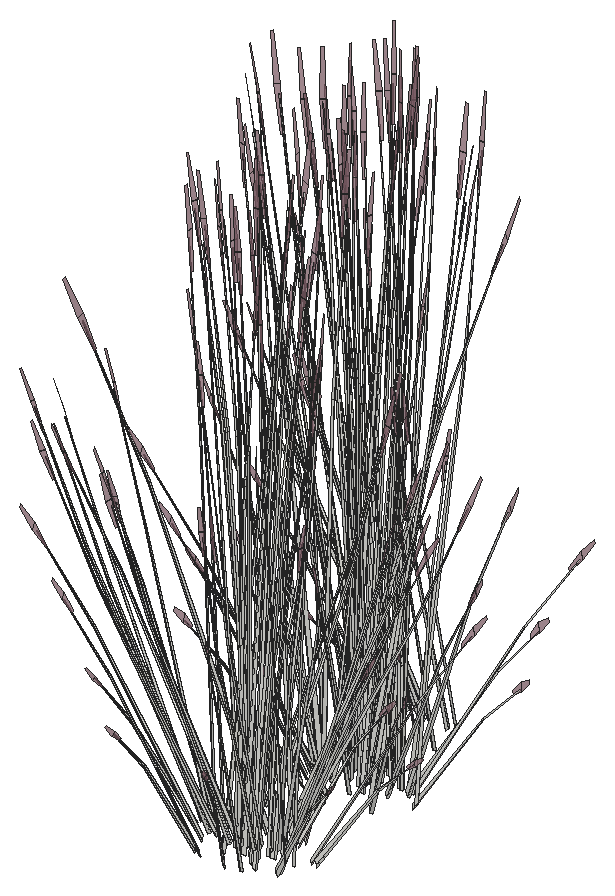
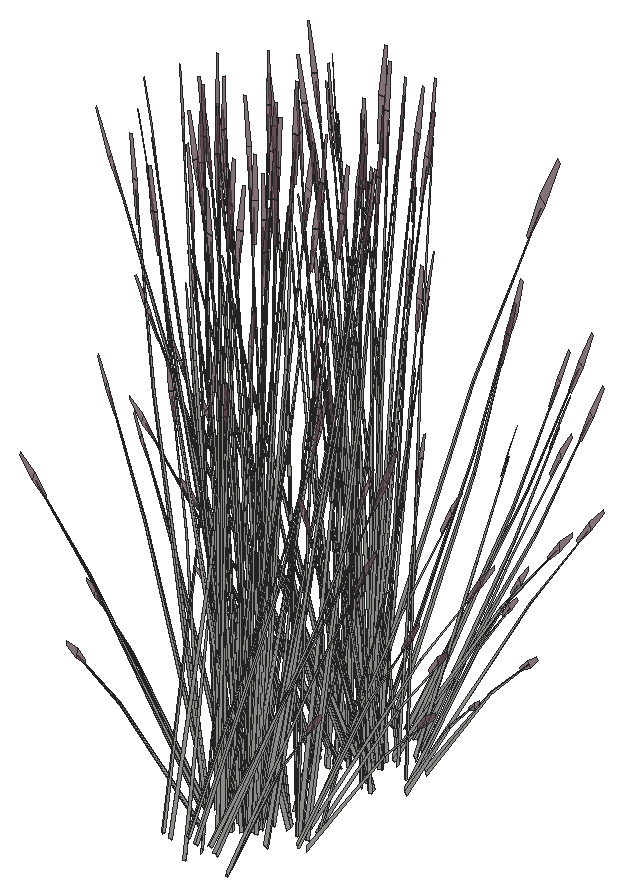
# SketchUp Ruby script. Lengths in inches.
U = 1.inch
M = Sketchup.active_model
def pt(a) = Geom::Point3d.new(a.map { |v| v * U })
def face(e, loops, mat)
  f = e.add_face(loops[0].map { |a| pt(a) })
  loops[1..].each { |l| e.add_face(l.map { |a| pt(a) }).erase! }
  f.material = f.back_material = mat if mat
  f
end
# faces: each face lists its corners as indices into pts; further lists are holes
def faces(e, pts, list, mat = nil) = list.each { |f| face(e, (f[0].is_a?(Array) ? f : [f]).map { |l| l.map { |i| pts[i] } }, mat) }
# xy, xz, yz: faces in a plane at the given z, y or x. An outline is a flat list of corners, or four numbers for a rectangle; further outlines are holes
def ring(l) = l.size == 4 ? [[l[0], l[1]], [l[2], l[1]], [l[2], l[3]], [l[0], l[3]]] : l.each_slice(2).to_a
def flat(e, list, mat, &to3) = list.each { |f| face(e, (f[0].is_a?(Array) ? f : [f]).map { |l| ring(l).map { |u, v| to3.(u, v) } }, mat) }
def xy(e, z, list, mat = nil) = flat(e, list, mat) { |x, y| [x, y, z] }
def xz(e, y, list, mat = nil) = flat(e, list, mat) { |x, z| [x, y, z] }
def yz(e, x, list, mat = nil) = flat(e, list, mat) { |y, z| [x, y, z] }
def lines(e, pts, list) = list.each { |a, b| e.add_line(pt(pts[a]), pt(pts[b])) }
# prism: a flat outline (further loops are holes) pulled along v
def prism(e, loops, v, mat = nil)
  f = face(e, loops, mat); d = Geom::Vector3d.new(v.map { |x| x * U })
  f.pushpull(f.normal.samedirection?(d) ? d.length : -d.length)
end
def box(e, o, s, mat = nil) = prism(e, [[o, [o[0] + s[0], o[1], o[2]], [o[0] + s[0], o[1] + s[1], o[2]], [o[0], o[1] + s[1], o[2]]]], [0, 0, s[2]], mat)
def at(x, y, z, deg = 0) = Geom::Transformation.translation(pt([x, y, z])) * Geom::Transformation.rotation(ORIGIN, Z_AXIS, deg.degrees)
def axes(o, x, y, z) = Geom::Transformation.new([*x, 0, *y, 0, *z, 0, *pt(o).to_a, 1])
def part(name) = M.definitions.add(name)
# library, detail: a bought-in or finely detailed component or shape, given as its bounding box
def library(name, o, s) = part(name).tap { |d| box(d.entities, o, s) }
def detail(e, o, s) = box(e.add_group.entities, o, s)
def put(e, d, t, mat = nil) = e.add_instance(d, t).tap { |i| i.material = mat if mat }
def group(e, t, mat = nil) = e.add_group.tap { |g| g.transformation = t; g.material = mat if mat }.entities
root = M.entities
M.materials.add("LightPink_Translucent").color = [144, 107, 117]
M.materials["LightPink_Translucent"].alpha = 0.75
c1 = part("blade")
p = [[2.15,0.21,22],[0,0.17,0],[0.09,0.45,0],[2.18,0.31,22],[2.29,0.31,22],[0.38,0.45,0],
  [2.48,0.24,33],[2.49,0.24,33],[2.48,0.22,33]]
faces(c1.entities,p,[[0,1,2,3],[4,5,2,3],[6,3,4,7],[8,0,3,6]])
c2 = part("seeds")
p = [[0.3,-0.1,1.38],[-0.01,-0.03,1.59],[-0.01,-0.03,0.03],[0.14,-0.07,-0.07],[0.29,-0.03,3],[0.15,0.01,3.11]]
faces(c2.entities,p,[[0,1,2,3],[1,0,4,5]],"LightPink_Translucent")
c3 = part("blade with seeds")
put(c3.entities,c1,at(0,0,0))
put(c3.entities,c2,axes([2.4,0.25,30.99],[1.5799,-0.05474,1.17369],[-0.12525,1.92788,0.29478],[-0.07173,-0.02425,1.56792]))
put(root,c3,axes([274.1,321.38,124.7],[-0.25429,0.13207,1.43002],[-0.76157,-0.23115,-0.30754],[0.14117,-0.28747,0.61141]))
put(root,c3,axes([272.94,321.84,127.09],[-0.42698,-0.53052,-0.71045],[0.87893,-0.29566,0.08574],[-0.09984,-0.25633,1.00501]))
put(root,c3,axes([270.16,321.13,124.7],[-0.05417,0.21344,1.43002],[-0.79196,0.17867,-0.30754],[-0.18512,-0.27588,0.61141]))
put(root,c3,axes([274.72,322.36,127.09],[0.02328,-0.60353,-0.71045],[0.98022,0.04053,0.08574],[0.10344,-0.25568,1.00501]))
put(root,c3,axes([272.62,321.73,126.79],[-0.87941,-0.16356,-0.51099],[0.30143,-0.56078,-0.3958],[-0.08064,-0.22578,0.97773]))
put(root,c3,axes([273.16,320.33,124.87],[0.11476,0.38047,1.1486],[-0.63664,-0.21072,0.84392],[0.06851,-0.19481,0.25299]))
put(root,c3,axes([274.52,322.16,126.79],[-0.64041,-0.4384,-0.51099],[0.67652,-0.38394,-0.3958],[0.09744,-0.22274,0.97773]))
put(root,c3,axes([269.89,320.79,124.87],[0.46666,0.22709,1.1486],[-0.67962,0.13651,0.84392],[-0.14541,-0.17452,0.25299]))
put(root,c3,axes([271.02,321.99,127.09],[-0.76283,-0.31537,-0.71045],[0.54213,-0.55263,0.08574],[-0.27638,-0.1883,1.00501]))
put(root,c3,axes([270.66,322.01,126.79],[-0.88277,0.1551,-0.51099],[-0.15442,-0.58737,-0.3958],[-0.23711,-0.16832,0.97773]))
put(root,c3,axes([275.875,323.41,127.09],[0.4673,-0.51481,-0.71045],[0.81887,0.36587,0.08574],[0.27902,-0.18652,1.00501]))
put(root,c3,axes([275.85,323.17,126.79],[-0.22982,-0.59576,-0.51099],[0.87033,-0.10422,-0.3958],[0.24941,-0.16002,0.97773]))
put(root,c3,axes([272.84,325.56,125.43],[0.77308,0.2631,1.51261],[-0.75736,0.56681,0.59816],[-0.33924,-0.33594,1.26806]))
put(root,c3,axes([276.55,322.9375,124.7],[-0.31959,-0.01933,1.43002],[-0.32741,-0.51843,-0.30754],[0.39262,-0.14666,0.61141]))
put(root,c3,axes([276.92,321.98,124.87],[-0.29798,0.33213,1.1486],[-0.25612,-0.44624,0.84392],[0.24611,-0.11182,0.25299]))
put(root,c3,axes([268.74,322.93,124.7],[0.17466,0.18165,1.43002],[-0.40248,0.49377,-0.30754],[-0.41327,-0.11802,0.61141]))
put(root,c3,axes([269.46,322.77,127.09],[-0.89428,-0.01571,-0.71045],[0.06006,-0.66153,0.08574],[-0.37886,-0.06981,1.00501]))
put(root,c3,axes([272.0625,324.3,124.54],[1.00799,0.31623,0.24065],[-0.48511,0.65709,0.50002],[0,-0.15147,1.60543]))
put(root,c3,axes([269.17,322.9,126.79],[-0.6496,0.4322,-0.51099],[-0.5689,-0.45657,-0.3958],[-0.33005,-0.06576,0.97773]))
put(root,c3,axes([267.7,323.48,124.87],[0.57115,-0.04669,1.1486],[-0.36229,0.41137,0.84392],[-0.28224,-0.06171,0.25299]))
put(root,c3,axes([271.74,323.86,124.83],[-0.97146,0.04028,0.44739],[-0.08785,-0.66859,-0.21531],[0.17391,-0.06776,1.43643]))
put(root,c3,axes([269.23,324.35,124.59],[0,0.65246,0.49651],[-1.00089,0,0],[0,-0.1486,1.57504]))
put(root,c3,axes([276.26,324.49,126.79],[0.24236,-0.59349,-0.51099],[0.83094,0.20343,-0.3958],[0.33455,-0.05442,0.97773]))
put(root,c3,axes([271.7,324.1,124.47],[0.38895,0.72959,0.45755],[-1.11135,0.2537,0.17955],[0.01358,-0.13406,1.58856]))
put(root,c3,axes([271.51,324.67,124.83],[-0.43405,0.58792,0.44739],[-0.90188,-0.28295,-0.21531],[0,-0.13553,1.43643]))
put(root,c3,axes([274.46,322.42,124.59],[-0.83726,-0.32623,0.49651],[0.50045,-0.58498,0],[0.19069,0.0743,1.57504]))
put(root,c3,axes([276.1,324.71,127.09],[0.78611,-0.28816,-0.71045],[0.4381,0.59317,0.08574],[0.37982,-0.06738,1.00501]))
put(root,c3,axes([272.57,323.68,124.47],[-0.74176,0.59212,0.45755],[-0.88124,-0.52269,0.17955],[0.17882,-0.05909,1.58856]))
put(root,c3,axes([271.29,322.71,124.58],[-0.25843,0.64844,0.17642],[-0.9457,-0.1835,0.35086],[0.16336,-0.00316,1.60407]))
put(root,c3,axes([273.26,323.43,124.72],[0.17258,-0.58229,0.1448],[0.84319,0.10108,-0.41347],[0.15345,0.05979,1.26744]))
put(root,c3,axes([271.8,324.8125,124.47],[1.13071,0.13747,0.45755],[-0.23011,0.77639,0.17955],[-0.16524,-0.07497,1.58856]))
put(root,c3,axes([272.9,323.58,124.83],[-0.53742,-0.54764,0.44739],[0.81403,-0.38564,-0.21531],[0.17391,0.06776,1.43643]))
put(root,c3,axes([271.19,326.05,124.58],[0.96132,-0.17317,0.17642],[0.23737,0.64447,0.35086],[-0.08574,-0.0939,1.60407]))
put(root,c3,axes([274.15,322.75,124.58],[-0.96132,0.17317,0.17642],[-0.23737,-0.64447,0.35086],[0.08574,0.0939,1.60407]))
put(root,c3,axes([273.54,323.99,124.49],[-1.13071,-0.13747,0.49198],[0.23011,-0.77639,0.19306],[0.16524,0.07497,1.70813]))
put(root,c3,axes([272.08,325.37,124.72],[-0.17258,0.58229,0.1448],[-0.84319,-0.10108,-0.41347],[-0.15345,-0.05979,1.26744]))
put(root,c3,axes([274.05,326.09,124.58],[0.25843,-0.64844,0.17642],[0.9457,0.1835,0.35086],[-0.16336,0.00316,1.60407]))
put(root,c3,axes([270.29,323.83,125.45],[0.25429,-0.09438,1.77064],[0.08769,0.65901,0.13857],[-0.5508,0.08745,0.63284]))
put(root,c3,axes([275.53,324.44,124.58],[-0.70288,-0.47526,0.17642],[0.70832,-0.46097,0.35086],[-0.07763,0.09706,1.60407]))
put(root,c3,axes([278.34,324.87,124.87],[-0.55274,0.10771,1.1486],[0.26018,-0.44517,0.84392],[0.29323,0.03046,0.25299]))
put(root,c3,axes([270.88,326.38,124.59],[0.83726,0.32623,0.49651],[-0.50045,0.58498,0],[-0.19069,-0.0743,1.57504]))
put(root,c3,axes([273.83,324.125,124.83],[0.43405,-0.58792,0.44739],[0.90188,0.28295,-0.21531],[0,0.13553,1.43643]))
put(root,c3,axes([268.54,324.1875,126.79],[-0.24236,0.59349,-0.51099],[-0.83094,-0.20343,-0.3958],[-0.33455,0.05442,0.97773]))
put(root,c3,axes([276.11,324.45,124.59],[0,-0.65246,0.49651],[1.00089,0,0],[0,0.1486,1.57504]))
put(root,c3,axes([273.6,324.94,124.83],[0.97146,-0.04028,0.44739],[0.08785,0.66859,-0.21531],[-0.17391,0.06776,1.43643]))
put(root,c3,axes([274.21,324.26,124.72],[0.83351,-0.19028,0.1448],[0.29189,0.54335,-0.41347],[0,0.11958,1.26744]))
put(root,c3,axes([277.31,325.58,124.7],[-0.21545,-0.16047,1.43002],[0.28033,-0.53085,-0.30754],[0.43591,0.07191,0.61141]))
put(root,c3,axes([273.62,325.23,124.72],[0.66093,0.39201,0.1448],[-0.5513,0.44227,-0.41347],[-0.15345,0.05979,1.26744]))
put(root,c3,axes([275.33,325.91,127.09],[0.89428,0.01571,-0.71045],[-0.06006,0.66153,0.08574],[0.37886,0.06981,1.00501]))
put(root,c3,axes([274.32,326.4375,124.59],[0.83726,-0.32623,0.49651],[0.50045,0.58498,0],[-0.19069,0.0743,1.57504]))
put(root,c3,axes([267.54,325.58,124.7],[0.3109,0.05356,1.43002],[0.20038,0.54709,-0.30754],[-0.42231,0.10241,0.61141]))
put(root,c3,axes([266.89,326.73,124.87],[0.37283,-0.29571,1.1486],[0.14711,0.46813,0.84392],[-0.26943,0.08382,0.25299]))
put(root,c3,axes([275.27,326.41,124.87],[-0.5037,-0.18761,1.1486],[0.6504,-0.19062,0.84392],[0.17543,0.16147,0.25299]))
put(root,c3,axes([268.94,325.51,126.79],[0.22982,0.59576,-0.51099],[-0.87033,0.10422,-0.3958],[-0.24941,0.16002,0.97773]))
put(root,c3,axes([274.1,334.36,125.6],[-0.25429,0.13207,1.43002],[-0.76157,-0.23115,-0.30754],[0.14117,-0.28747,0.61141]))
put(root,c3,axes([270.16,334.11,125.6],[-0.05417,0.21344,1.43002],[-0.79196,0.17867,-0.30754],[-0.18512,-0.27588,0.61141]))
put(root,c3,axes([274.04,324.3,124.95],[-0.02444,-0.61432,1.41272],[1.10603,0.15924,0.59816],[-0.26159,0.33615,1.3335]))
put(root,c3,axes([274.13,326.67,126.79],[0.88277,-0.1551,-0.51099],[0.15442,0.58737,-0.3958],[0.23711,0.16832,0.97773]))
put(root,c3,axes([272.2,333.64,124.51],[-0.15005,0.02351,1.76342],[-0.82981,-0.26461,-0.26939],[0.01392,-0.22072,0.30037]))
put(root,c3,axes([275.35,327.27,124.77],[-0.57368,-0.02046,1.0506],[0.37886,-0.43461,0.58006],[0.22663,0.15441,0.8241]))
put(root,c3,axes([273.48,326.21,124.7],[0.01579,-0.21629,1.43002],[0.75442,-0.24159,-0.30754],[0.23289,0.25887,0.61141]))
put(root,c3,axes([270.05,328.02,124.87],[-0.02315,-0.38796,1.1486],[0.57853,0.27671,0.84392],[-0.11378,0.18492,0.25299]))
put(root,c3,axes([270.27,326.52,127.11],[0.64041,0.4384,-0.5672],[-0.67652,0.38394,-0.43934],[-0.09744,0.22274,1.08528]))
put(root,c3,axes([269.57,327.18,124.93],[0.8127,-0.11554,0.06507],[0.18684,0.46549,-0.86304],[-0.05152,0.23564,0.7736]))
put(root,c3,axes([272.17,326.94,126.79],[0.87941,0.16356,-0.51099],[-0.30143,0.56078,-0.3958],[0.08064,0.22578,0.97773]))
put(root,c3,axes([269.52,334.45,124.51],[-0.08666,0.08595,1.76342],[-0.87574,0.18531,-0.26939],[-0.21156,-0.16858,0.30037]))
put(root,c3,axes([275.88,334.77,124.51],[-0.1339,-0.0514,1.76342],[-0.34394,-0.57425,-0.26939],[0.23202,-0.15583,0.30037]))
put(root,c3,axes([270.07,326.32,127.45],[-0.02328,0.60353,-0.7886],[-0.98022,-0.04053,0.09517],[-0.10344,0.25568,1.11556]))
put(root,c3,axes([271.85,326.84,127.09],[0.42698,0.53052,-0.71045],[-0.87893,0.29566,0.08574],[0.09984,0.25633,1.00501]))
put(root,c3,axes([270.82,334.89,125.39],[-0.55932,-0.6538,0],[0.93577,-0.36461,-0.51607],[0.21313,-0.08304,1.63711]))
put(root,c3,axes([269.38,327.67,124.7],[0.28231,-0.10293,1.43002],[0.69701,0.31035,-0.30754],[-0.20746,0.26854,0.61141]))
put(root,c3,axes([272.05,334.1,125.14],[-0.61821,0.37431,-0.03893],[-0.56645,-0.40995,-0.17649],[-0.03988,-0.11616,0.58215]))
put(root,c3,axes([276.55,335.91,125.6],[-0.31959,-0.01933,1.43002],[-0.32741,-0.51843,-0.30754],[0.39262,-0.14666,0.61141]))
put(root,c3,axes([269.74,327.17,125.47],[0.01966,-0.33682,1.54345],[0.88405,0.17791,0.21329],[-0.0766,0.35897,0.72882]))
put(root,c3,axes([271.92,336.69,125.68],[-0.10425,-0.7445,-0.29095],[1.08575,-0.04502,-0.50002],[0.19119,-0.09917,1.59708]))
put(root,c3,axes([268.98,334.78,125.14],[-0.25807,0.53277,-0.03893],[-0.79428,-0.16389,-0.17649],[-0.1206,-0.08714,0.58215]))
put(root,c3,axes([271.42,337.47,125.68],[-1.00749,-0.31132,-0.29095],[0.48511,-0.65709,-0.50002],[-0.03166,-0.16133,1.59708]))
put(root,c3,axes([268.55,337.21,125.39],[-1.11865,0,0],[0,-0.72922,-0.51607],[0,-0.16609,1.63711]))
put(root,c3,axes([268.74,335.91,125.6],[0.17466,0.18165,1.43002],[-0.40248,0.49377,-0.30754],[-0.41327,-0.11802,0.61141]))
put(root,c3,axes([269.42,337.02,125.34],[-0.83213,0.54855,0.30756],[-0.83263,-0.54278,-0.36492],[-0.02906,-0.15578,1.64885]))
put(root,c3,axes([272.0625,337.28,125.45],[1.00799,0.31623,0.24065],[-0.48511,0.65709,0.50002],[0,-0.15147,1.60543]))
put(root,c3,axes([271.67,338.16,125.45],[0.23711,-0.77313,-0.23429],[1.12425,0.13477,0.51271],[-0.19645,-0.10677,1.5644]))
put(root,c3,axes([269.23,337.32,125.49],[0,0.65246,0.49651],[-1.00089,0,0],[0,-0.1486,1.57504]))
put(root,c3,axes([274.94,335.05,125.39],[0.55932,-0.6538,0],[0.93577,0.36461,-0.51607],[0.21313,0.08304,1.63711]))
put(root,c3,axes([271.7,337.08,125.375],[0.38895,0.72959,0.45755],[-1.11135,0.2537,0.17955],[0.01358,-0.13406,1.58856]))
put(root,c3,axes([277.14,337.64,125],[-0.57619,0.0783,1.41583],[-0.09171,-0.62326,0.08104],[0.40356,-0.09434,0.80566]))
put(root,c3,axes([278.19,337.08,125.27],[-0.55463,-0.41721,-0.06488],[0.60744,-0.38228,-0.29416],[0.17212,-0.02691,0.97024]))
put(root,c3,axes([273.1,337.14,125.22],[0,-0.75495,0],[1.11865,0,0],[0,0,1.79456]))
put(root,c3,axes([274.46,335.39,125.49],[-0.83726,-0.32623,0.49651],[0.50045,-0.58498,0],[0.19069,0.0743,1.57504]))
put(root,c3,axes([272.57,336.66,125.375],[-0.74176,0.59212,0.45755],[-0.88124,-0.52269,0.17955],[0.17882,-0.05909,1.58856]))
put(root,c3,axes([273.38,337.72,125.3125],[-0.83213,-0.56158,-0.06131],[0.83263,-0.56193,0],[-0.02906,-0.01961,1.75571]))
put(root,c3,axes([271.29,335.6875,125.49],[-0.25843,0.64844,0.17642],[-0.9457,-0.1835,0.35086],[0.16336,-0.00316,1.60407]))
put(root,c3,axes([270.89,336.21,124.61],[-0.88056,0.26122,1.28929],[-0.28027,-0.74951,0.50096],[0.54072,0.01247,1.46642]))
put(root,c3,axes([273.26,336.41,125.63],[0.17258,-0.58229,0.1448],[0.84319,0.10108,-0.41347],[0.15345,0.05979,1.26744]))
put(root,c3,axes([271.8,337.79,125.375],[1.13071,0.13747,0.45755],[-0.23011,0.77639,0.17955],[-0.16524,-0.07497,1.58856]))
put(root,c3,axes([277.77,337.23,124.51],[-0.04675,-0.09906,1.76342],[0.32428,-0.57943,-0.26939],[0.32711,-0.00833,0.30037]))
put(root,c3,axes([268.12,337.125,124.51],[0.02269,0.10283,1.76342],[-0.45738,0.53699,-0.26939],[-0.32488,-0.02707,0.30037]))
put(root,c3,axes([271.19,339.03,125.49],[0.96132,-0.17317,0.17642],[0.23737,0.64447,0.35086],[-0.08574,-0.0939,1.60407]))
put(root,c3,axes([273.17,336.6,125.68],[0.90324,-0.43318,-0.29095],[0.60064,0.61207,-0.50002],[0.22285,0.06216,1.59708]))
put(root,c3,axes([273.86,337.31,125.22],[1.00089,0,0],[0,0.67548,0],[0,0,1.78407]))
put(root,c3,axes([272.17,338.16,125.68],[-0.90324,0.43318,-0.29095],[-0.60064,-0.61207,-0.50002],[-0.22285,-0.06216,1.59708]))
put(root,c3,axes([274.15,335.72,125.49],[-0.96132,0.17317,0.17642],[-0.23737,-0.64447,0.35086],[0.08574,0.0939,1.60407]))
put(root,c3,axes([273.54,336.96,125.39],[-1.13071,-0.13747,0.49198],[0.23011,-0.77639,0.19306],[0.16524,0.07497,1.70813]))
put(root,c3,axes([272.64,338.88,125.22],[-0.29189,-0.56252,0],[0.83351,-0.19699,0],[0,0,1.54371]))
put(root,c3,axes([272.08,338.35,125.63],[-0.17258,0.58229,0.1448],[-0.84319,-0.10108,-0.41347],[-0.15345,-0.05979,1.26744]))
put(root,c3,axes([273.73,338.8,125.2],[0.93921,-0.22138,-0.19198],[0.33003,0.6377,0.00008],[0.10367,-0.02447,1.73897]))
put(root,c3,axes([274.05,339.07,125.49],[0.25843,-0.64844,0.17642],[0.9457,0.1835,0.35086],[-0.16336,0.00316,1.60407]))
put(root,c3,axes([273.84,337.6,125.23],[0.62448,0.42144,0],[-0.62448,0.42144,0],[0,0,1.69266]))
put(root,c3,axes([275.53,337.41,125.49],[-0.70288,-0.47526,0.17642],[0.70832,-0.46097,0.35086],[-0.07763,0.09706,1.60407]))
put(root,c3,axes([272.43,339.13,125.21],[-0.90188,-0.29293,0],[0.43405,-0.60866,0],[0,0,1.62707]))
put(root,c3,axes([273.18,338.35,125.48],[-0.87356,-0.52515,-0.25192],[0.73507,-0.5897,0.5513],[-0.23523,0.06143,1.68216]))
put(root,c3,axes([273.67,337.4375,125.31],[0,0.75458,-0.05637],[-1.11865,0,0],[0,0.02371,1.79368]))
put(root,c3,axes([270.4,339.7,125.39],[-0.55932,0.6538,0],[-0.93577,-0.36461,-0.51607],[-0.21313,-0.08304,1.63711]))
put(root,c3,axes([276.11,337.43,125.49],[0,-0.65246,0.49651],[1.00089,0,0],[0,0.1486,1.57504]))
put(root,c3,axes([274.21,337.24,125.63],[0.83351,-0.19028,0.1448],[0.29189,0.54335,-0.41347],[0,0.11958,1.26744]))
put(root,c3,axes([277.31,338.5625,125.6],[-0.21545,-0.16047,1.43002],[0.28033,-0.53085,-0.30754],[0.43591,0.07191,0.61141]))
put(root,c3,axes([274.1,344.63,124.91],[-0.25429,0.13207,1.43002],[-0.76157,-0.23115,-0.30754],[0.14117,-0.28747,0.61141]))
put(root,c3,axes([272.94,345.09,127.3],[-0.42698,-0.53052,-0.71045],[0.87893,-0.29566,0.08574],[-0.09984,-0.25633,1.00501]))
put(root,c3,axes([273.45,339.14,125.22],[0.90188,0.29293,0],[-0.43405,0.60866,0],[0,0,1.74954]))
put(root,c3,axes([270.16,344.38,124.91],[-0.05417,0.21344,1.43002],[-0.79196,0.17867,-0.30754],[-0.18512,-0.27588,0.61141]))
put(root,c3,axes([273.8125,339.79,125.21],[-0.55235,-0.65609,-0.05142],[0.93577,-0.36461,0.51607],[-0.23059,0.06247,1.6363]))
put(root,c3,axes([273.62,338.21,125.63],[0.66093,0.39201,0.1448],[-0.5513,0.44227,-0.41347],[-0.15345,0.05979,1.26744]))
put(root,c3,axes([274.72,345.61,127.3],[0.02328,-0.60353,-0.71045],[0.98022,0.04053,0.08574],[0.10344,-0.25568,1.00501]))
put(root,c3,axes([273.13,338.9,125.3],[0.38895,0.74956,-0.06012],[-1.11135,0.26265,0],[0.01358,0.02618,1.72173]))
put(root,c3,axes([272.62,344.99,127],[-0.87941,-0.16356,-0.51099],[0.30143,-0.56078,-0.3958],[-0.08064,-0.22578,0.97773]))
put(root,c3,axes([273.16,343.58,125.09],[0.11476,0.38047,1.1486],[-0.63664,-0.21072,0.84392],[0.06851,-0.19481,0.25299]))
put(root,c3,axes([267.54,338.56,125.6],[0.3109,0.05356,1.43002],[0.20038,0.54709,-0.30754],[-0.42231,0.10241,0.61141]))
put(root,c3,axes([274.52,345.41,127],[-0.64041,-0.4384,-0.51099],[0.67652,-0.38394,-0.3958],[0.09744,-0.22274,0.97773]))
put(root,c3,axes([276.79,337.54,125.39],[1.11865,0,0],[0,0.72922,-0.51607],[0,0.16609,1.63711]))
put(root,c3,axes([276.34,337.92,125.21],[-1.1181,-0.00522,-0.04976],[0,-0.72922,0.49943],[-0.03514,0.166,1.58352]))
put(root,c3,axes([273.92,337.28,125.68],[1.00749,0.31132,-0.29095],[-0.48511,0.65709,-0.50002],[0.03166,0.16133,1.59708]))
put(root,c3,axes([273.42,338.0625,125.68],[0.10425,0.7445,-0.29095],[-1.08575,0.04502,-0.50002],[-0.19119,0.09917,1.59708]))
put(root,c3,axes([269.89,344.04,125.09],[0.46666,0.22709,1.1486],[-0.67962,0.13651,0.84392],[-0.14541,-0.17452,0.25299]))
put(root,c3,axes([271.02,345.24,127.3],[-0.76283,-0.31537,-0.71045],[0.54213,-0.55263,0.08574],[-0.27638,-0.1883,1.00501]))
put(root,c3,axes([273.84,339.46,125.34],[1.11998,0.21207,0.30756],[-0.2802,0.75803,-0.36492],[-0.18537,0.09487,1.64885]))
put(root,c3,axes([270.66,345.26,127],[-0.88277,0.1551,-0.51099],[-0.15442,-0.58737,-0.3958],[-0.23711,-0.16832,0.97773]))
put(root,c3,axes([274.52,339.87,125.39],[0.55932,0.6538,0],[-0.93577,0.36461,-0.51607],[-0.21313,0.08304,1.63711]))
put(root,c3,axes([275.41,340.09,124.51],[0.06518,-0.0942,1.76342],[0.82057,-0.27742,-0.26939],[0.24877,0.14358,0.30037]))
